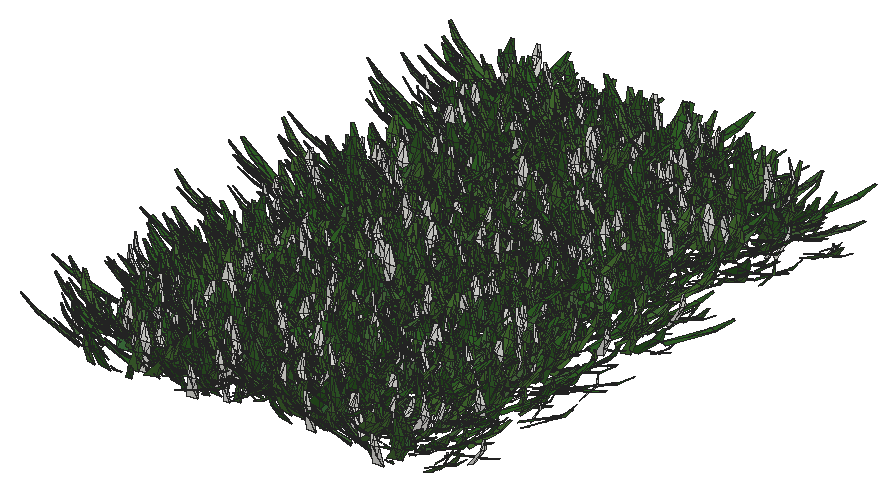
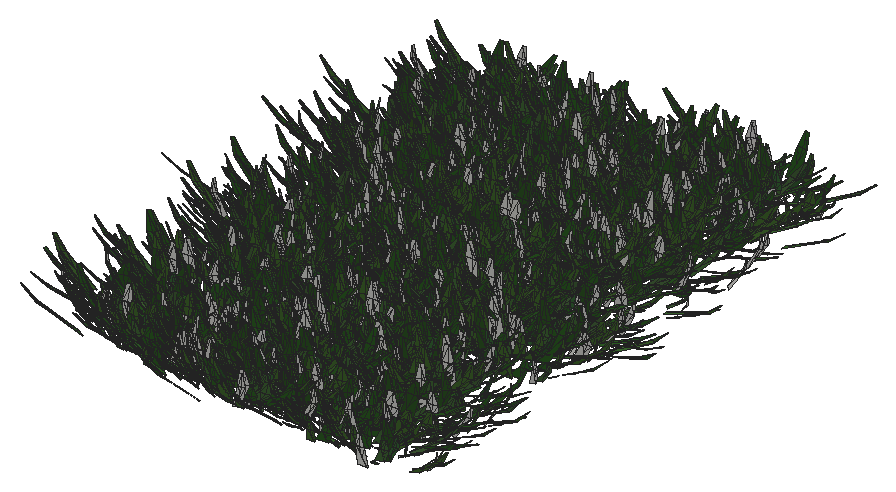
# SketchUp Ruby script. Lengths in inches.
U = 1.inch
M = Sketchup.active_model
def pt(a) = Geom::Point3d.new(a.map { |v| v * U })
def face(e, loops, mat)
  f = e.add_face(loops[0].map { |a| pt(a) })
  loops[1..].each { |l| e.add_face(l.map { |a| pt(a) }).erase! }
  f.material = f.back_material = mat if mat
  f
end
# faces: each face lists its corners as indices into pts; further lists are holes
def faces(e, pts, list, mat = nil) = list.each { |f| face(e, (f[0].is_a?(Array) ? f : [f]).map { |l| l.map { |i| pts[i] } }, mat) }
# xy, xz, yz: faces in a plane at the given z, y or x. An outline is a flat list of corners, or four numbers for a rectangle; further outlines are holes
def ring(l) = l.size == 4 ? [[l[0], l[1]], [l[2], l[1]], [l[2], l[3]], [l[0], l[3]]] : l.each_slice(2).to_a
def flat(e, list, mat, &to3) = list.each { |f| face(e, (f[0].is_a?(Array) ? f : [f]).map { |l| ring(l).map { |u, v| to3.(u, v) } }, mat) }
def xy(e, z, list, mat = nil) = flat(e, list, mat) { |x, y| [x, y, z] }
def xz(e, y, list, mat = nil) = flat(e, list, mat) { |x, z| [x, y, z] }
def yz(e, x, list, mat = nil) = flat(e, list, mat) { |y, z| [x, y, z] }
def lines(e, pts, list) = list.each { |a, b| e.add_line(pt(pts[a]), pt(pts[b])) }
# prism: a flat outline (further loops are holes) pulled along v
def prism(e, loops, v, mat = nil)
  f = face(e, loops, mat); d = Geom::Vector3d.new(v.map { |x| x * U })
  f.pushpull(f.normal.samedirection?(d) ? d.length : -d.length)
end
def box(e, o, s, mat = nil) = prism(e, [[o, [o[0] + s[0], o[1], o[2]], [o[0] + s[0], o[1] + s[1], o[2]], [o[0], o[1] + s[1], o[2]]]], [0, 0, s[2]], mat)
def at(x, y, z, deg = 0) = Geom::Transformation.translation(pt([x, y, z])) * Geom::Transformation.rotation(ORIGIN, Z_AXIS, deg.degrees)
def axes(o, x, y, z) = Geom::Transformation.new([*x, 0, *y, 0, *z, 0, *pt(o).to_a, 1])
def part(name) = M.definitions.add(name)
# library, detail: a bought-in or finely detailed component or shape, given as its bounding box
def library(name, o, s) = part(name).tap { |d| box(d.entities, o, s) }
def detail(e, o, s) = box(e.add_group.entities, o, s)
def put(e, d, t, mat = nil) = e.add_instance(d, t).tap { |i| i.material = mat if mat }
def group(e, t, mat = nil) = e.add_group.tap { |g| g.transformation = t; g.material = mat if mat }.entities
root = M.entities
M.materials.add("Material82").color = [68, 110, 58]
M.materials.add("Material83").color = [48, 90, 38]
M.materials.add("Material84").color = [68, 110, 48]
M.materials.add("Material85").color = [48, 90, 48]
M.materials.add("Material86").color = [58, 110, 58]
M.materials.add("Material87").color = [58, 90, 38]
M.materials.add("Material88").color = [68, 100, 58]
M.materials.add("Material89").color = [48, 100, 38]
c1 = part("grass00")
p = [[-0.6875,0.15,0],[-0.56,0.08,5.52],[-0.04,0.03,2.76],[0.48,-0.02,0],[0.35,-0.02,5.52],[-0.1,-0.14,5.52],
  [-0.12,0.65,8.37],[-0.42,0.65,8.37]]
faces(c1.entities,p,[[0,1,2,3],[3,2,4],[1,5,2],[5,4,2],[1,6,5],[4,5,6],[7,6,1]])
c2 = part("Group16\#1")
put(c2.entities,c1,axes([1.44,-0.61,-0.01],[0.05352,0.12609,0],[-0.10704,0.04543,0.07239],[0.06664,-0.02828,0.11628]),"Material85")
put(c2.entities,c1,axes([0.76,-0.15,-0.01],[0.04676,0.24062,0],[-0.23162,0.04501,0.06642],[0.0652,-0.01267,0.23595]),"Material82")
put(c2.entities,c1,axes([0.79,0.01,-0.01],[-0.00606,0.34651,0],[-0.34381,-0.00602,0.0432],[0.04319,0.00076,0.34386]))
put(c2.entities,c1,axes([1,0.23,-0.01],[-0.07192,0.31144,0],[-0.28722,-0.06632,0.1236],[0.12043,0.02781,0.29478]),"Material84")
put(c2.entities,c1,axes([1.66,0.77,-0.01],[-0.13828,0.29651,0],[-0.21551,-0.1005,0.22471],[0.20365,0.09498,0.23779]),"Material89")
put(c2.entities,c1,axes([0.6875,0.52,-0.01],[-0.18126,0.24051,0],[-0.22746,-0.17142,0.09788],[0.07817,0.05891,0.28481]),"Material84")
put(c2.entities,c1,axes([0.68,0.78,-0.01],[-0.215,0.18688,0],[-0.12385,-0.14248,0.21334],[0.13995,0.16101,0.18878]),"Material82")
put(c2.entities,c1,axes([0.56,1,-0.01],[-0.13756,0.07624,0],[-0.06159,-0.11112,0.0927],[0.04494,0.08108,0.12705]),"Material84")
put(c2.entities,c1,axes([0.2,0.64,-0.01],[-0.23729,0.07254,0],[-0.05711,-0.18681,0.153],[0.04473,0.14632,0.19535]),"Material89")
put(c2.entities,c1,axes([0.0625,0.72,-0.01],[-0.28874,0.02525,0],[-0.02179,-0.24916,0.14647],[0.01276,0.14591,0.25012]),"Material82")
put(c2.entities,c1,axes([-0.08,0.62,-0.01],[-0.34089,-0.04187,0],[0.03255,-0.26504,0.216],[-0.02633,0.21439,0.26703]),"Material89")
put(c2.entities,c1,axes([-0.34,0.98,-0.01],[-0.14314,-0.0493,0],[0.04397,-0.12769,0.06843],[-0.02228,0.0647,0.13505]),"Material89")
put(c2.entities,c1,axes([-0.87,1.45,-0.01],[-0.23488,-0.14114,0],[0.13761,-0.22901,0.06087],[-0.03135,0.05217,0.26717]))
put(c2.entities,c1,axes([-0.72,0.77,-0.01],[-0.14208,-0.13251,0],[0.07209,-0.0773,0.16301],[-0.11118,0.11922,0.1057]),"Material89")
put(c2.entities,c1,axes([-0.62,0.43,-0.01],[-0.14845,-0.21203,0],[0.18654,-0.13061,0.12304],[-0.10079,0.07057,0.22772]),"Material82")
put(c2.entities,c1,axes([-0.68,0.29,-0.01],[-0.13639,-0.32136,0],[0.31723,-0.13464,0.05579],[-0.05136,0.0218,0.34462]),"Material83")
put(c2.entities,c1,axes([-0.64,0.125,-0.01],[-0.0458,-0.23569,0],[0.22124,-0.043,0.08276],[-0.08124,0.01579,0.22538]),"Material86")
put(c2.entities,c1,axes([-1.6,-0.03,-0.01],[0.00576,-0.32897,0],[0.27526,0.00482,0.18018],[-0.18015,-0.00315,0.2753]),"Material84")
put(c2.entities,c1,axes([-1.36,-0.31,-0.01],[0.05718,-0.24765,0],[0.18172,0.04196,0.17267],[-0.16825,-0.03885,0.1865]),"Material89")
put(c2.entities,c1,axes([-1.54,-0.72,-0.01],[0.06537,-0.14017,0],[0.13555,0.06321,0.03939],[-0.0357,-0.01665,0.14956]))
put(c2.entities,c1,axes([-1.19,-0.9,-0.01],[0.09597,-0.12735,0],[0.11214,0.08451,0.07557],[-0.06035,-0.04548,0.14042]),"Material88")
put(c2.entities,c1,axes([-0.47,-0.54,-0.01],[0.11588,-0.10072,0],[0.0618,0.0711,0.12124],[-0.07953,-0.0915,0.0942]))
put(c2.entities,c1,axes([-0.47,-0.84,-0.01],[0.11927,-0.0661,0],[0.06603,0.11913,0.00646],[-0.00313,-0.00565,0.13621]),"Material84")
put(c2.entities,c1,axes([-0.38,-1.24,-0.01],[0.28037,-0.08571,0],[0.0618,0.20215,0.20315],[-0.05939,-0.19428,0.21139]),"Material88")
put(c2.entities,c1,axes([-0.06,-0.66,-0.01],[0.22719,-0.01987,0],[0.01247,0.14255,0.17758],[-0.01547,-0.17691,0.1431]),"Material87")
put(c2.entities,c1,axes([0.11,-0.89,-0.01],[0.14882,0.01828,0],[-0.01058,0.08611,0.12229],[0.01491,-0.12138,0.08676]),"Material85")
put(c2.entities,c1,axes([0.25,-0.72,-0.01],[0.20481,0.07053,0],[-0.06206,0.18022,0.10291],[0.03351,-0.0973,0.1906]),"Material85")
put(c2.entities,c1,axes([0.85,-1.42,-0.01],[0.16481,0.09904,0],[-0.09472,0.15762,0.05616],[0.02893,-0.04814,0.18389]),"Material84")
put(c2.entities,c1,axes([1.01,-1.09,-0.01],[0.21858,0.20385,0],[-0.17495,0.1876,0.15339],[0.10462,-0.11218,0.25652]),"Material89")
put(c2.entities,c1,axes([1.01,-0.71,-0.01],[0.08733,0.12473,0],[-0.06445,0.04512,0.13037],[0.1068,-0.07477,0.07867]),"Material85")
c3 = part("Group15\#1")
put(c3.entities,c2,at(0,0,0))
c4 = part("3darcstudiotree_grass00\#1")
put(c4.entities,c3,at(0,0,0))
put(root,c4,axes([1826.34,333.52,-34.17],[0.25601,-1.60576,0],[3.7655,0.09337,-0.00515],[0.03185,0.00079,1.75106]))
put(root,c4,axes([1825.33,340.01,-34.17],[3.21046,-0.42194,0],[1.31397,1.55496,-0.01535],[0.02427,0.02872,1.5577]))
put(root,c4,axes([1825.35,312.04,-34.17],[-1.88352,1.24088,0],[-3.53635,-0.83485,-0.03562],[-0.13641,-0.0322,1.37892]))
put(root,c4,axes([1826.07,283.93,-34.17],[0.35251,-1.39793,0],[3.51175,0.13773,-0.03727],[0.24286,0.00952,1.73202]))
put(root,c4,axes([1826.34,289.67,-34.17],[-3.43821,0.20499,0],[-0.69374,-1.80975,-0.03474],[-0.02131,-0.0556,1.42794]))
put(root,c4,axes([1825.4,298.68,-34.17],[-0.07716,1.61232,0],[-4.08051,-0.03037,-0.05443],[-0.27918,-0.00208,1.56933]))
put(root,c4,axes([1826.95,320.22,-34.17],[1.28288,-1.22527,0],[4.05082,0.65965,-0.04448],[0.2416,0.03934,1.93016]))
put(root,c4,axes([1827.22,328.61,-34.17],[-0.2981,-1.54731,0],[4.18924,-0.12553,-0.05563],[0.33136,-0.00993,1.88098]))
put(root,c4,axes([1827.06,317.46,-34.17],[-0.54088,1.62044,0],[-3.31155,-0.17191,-0.03263],[-0.19335,-0.01004,1.49628]))
put(root,c4,axes([1827.25,315.92,-34.17],[3.70566,-0.42814,0],[1.15173,1.5504,-0.01036],[0.01836,0.02471,1.93559]))
put(root,c4,axes([1827.75,281.24,-34.17],[2.92691,-1.3802,0],[3.11862,1.02859,-0.02296],[0.10607,0.03499,1.8355]))
put(root,c4,axes([1828.3125,338.09,-34.17],[-3.14741,0.41412,0],[-1.12782,-1.33315,-0.01591],[-0.02767,-0.03271,1.46774]))
put(root,c4,axes([1827.55,335.22,-34.17],[-0.97344,1.33602,0],[-4.5066,-0.51069,-0.06106],[-0.24596,-0.02787,1.47293]))
put(root,c4,axes([1827.37,304.44,-34.17],[4.64499,-0.27977,0],[0.53132,1.372,-0.02943],[0.02555,0.06597,1.51666]))
put(root,c4,axes([1828.82,302.05,-34.17],[-0.18207,-1.50592,0],[4.09357,-0.07698,-0.05646],[0.28834,-0.00542,1.57058]))
put(root,c4,axes([1827.49,291.67,-34.17],[2.47814,1.17598,0],[-3.14029,1.02922,-0.05468],[-0.21842,0.07159,1.58958]))
put(root,c4,axes([1827.46,313.96,-34.17],[4.42055,0.62646,0],[-1.4719,1.61538,-0.03831],[-0.06085,0.06679,1.53223]))
put(root,c4,axes([1827.99,330.81,-34.17],[4.51641,-0.1704,0],[0.33815,1.39393,-0.00501],[0.00291,0.012,1.62495]))
put(root,c4,axes([1827.6875,293.85,-34.17],[2.33395,1.59128,0],[-3.69314,0.84246,-0.02506],[-0.12399,0.02828,1.82822]))
put(root,c4,axes([1828.27,285.62,-34.17],[3.72841,-0.11021,0],[0.34874,1.83494,-0.00347],[0.00143,0.00753,1.92949]))
put(root,c4,axes([1829.27,326.92,-34.17],[-2.15234,1.14546,0],[-3.3995,-0.99347,-0.05517],[-0.2418,-0.07066,1.72999]))
put(root,c4,axes([1828.57,300.64,-34.17],[2.3917,1.38211,0],[-2.775,0.74686,-0.01403],[-0.09111,0.02452,1.97952]))
put(root,c4,axes([1828.67,309.31,-34.17],[3.05644,0.96272,0],[-2.54771,1.25799,-0.04015],[-0.1144,0.05649,1.39698]))
put(root,c4,axes([1829.22,296.33,-34.17],[0.44258,1.4547,0],[-3.4051,0.16112,-0.01784],[-0.12417,0.00588,1.80168]))
put(root,c4,axes([1830.86,323.88,-34.17],[-1.45799,-1.43911,0],[3.11235,-0.49041,-0.01431],[0.09188,-0.01448,1.73701]))
put(root,c4,axes([1831.01,283.47,-34.17],[-2.77273,1.25915,0],[-2.61353,-0.89509,-0.01448],[-0.05898,-0.0202,1.39954]))
put(root,c4,axes([1831.98,285,-34.17],[-3.67224,-0.62774,0],[1.3268,-1.20717,-0.04544],[0.10775,-0.09803,1.4908]))
put(root,c4,axes([1832.23,317.6,-34.17],[-4.47177,0.4092,0],[-0.80597,-1.36984,-0.03599],[-0.04373,-0.07433,1.43677]))
put(root,c4,axes([1831.62,295.9,-34.17],[-3.07968,1.30519,0],[-3.32937,-1.22181,-0.01383],[-0.04412,-0.01619,1.48532]))
put(root,c4,axes([1832.39,339.19,-34.17],[-3.54635,0.32604,0],[-1.06041,-1.79388,-0.06463],[-0.05576,-0.09432,1.33032]))
put(root,c4,axes([1831.16,307.32,-34.17],[3.91717,0.58785,0],[-1.40512,1.45623,-0.01203],[-0.02325,0.0241,1.60927]))
put(root,c4,axes([1833.02,302.46,-34.17],[-1.04981,-1.26066,0],[3.51989,-0.45588,-0.02104],[0.10484,-0.01358,1.45661]))
put(root,c4,axes([1832.29,299.02,-34.17],[3.15172,-0.92963,0],[2.70365,1.42561,-0.02614],[0.06865,0.0362,1.48366]))
put(root,c4,axes([1833.06,305.26,-34.17],[-4.56421,0.17831,0],[-0.33265,-1.32435,-0.0174],[-0.0117,-0.04658,1.72585]))
put(root,c4,axes([1833.55,330.95,-34.17],[-3.08784,-0.53374,0],[1.78756,-1.6084,-0.00176],[0.00414,-0.00372,1.95594]))
put(root,c4,axes([1832.6,291.37,-34.17],[-2.14552,1.35971,0],[-3.80804,-0.93454,-0.04897],[-0.2422,-0.05944,1.9584]))
put(root,c4,axes([1832.0625,288.08,-34.17],[3.03533,0.518,0],[-1.31858,1.2017,-0.02703],[-0.08286,0.07551,1.9211]))
put(root,c4,axes([1833.9,313.28,-34.17],[-2.79081,-0.68685,0],[2.20267,-1.39196,-0.00523],[0.01654,-0.01045,1.86317]))
put(root,c4,axes([1834.04,316.69,-34.17],[-3.42781,-0.73376,0],[1.91044,-1.38806,-0.04387],[0.11882,-0.08633,1.70431]))
put(root,c4,axes([1833.34,289.42,-34.17],[-3.41152,0.77464,0],[-2.34689,-1.60751,-0.0199],[-0.0471,-0.03226,1.67187]))
put(root,c4,axes([1832.35,312.07,-34.17],[1.53269,1.16919,0],[-3.90157,0.79546,-0.03477],[-0.15934,0.03249,1.69826]))
put(root,c4,axes([1833.64,300.03,-34.17],[-2.82754,1.11661,0],[-2.90837,-1.14544,-0.05526],[-0.21558,-0.0849,1.69871]))
put(root,c4,axes([1833.65,293.44,-34.17],[2.39859,-1.38317,0],[2.89597,0.78107,-0.02882],[0.1286,0.03468,1.42183]))
put(root,c4,axes([1834.08,337.85,-34.17],[0.37671,-1.60669,0],[3.58296,0.13066,-0.04487],[0.23434,0.00855,1.41449]))
put(root,c4,axes([1834.48,336.35,-34.17],[-4.41181,-0.09171,0],[0.23476,-1.75641,-0.0488],[0.01273,-0.09527,1.65721]))
put(root,c4,axes([1834.35,281.67,-34.17],[-3.47293,0.19496,0],[-0.50842,-1.40863,-0.03826],[-0.03299,-0.09141,1.65468]))
put(root,c4,axes([1834.91,332.71,-34.17],[-4.2727,-0.29638,0],[0.78575,-1.76178,-0.04722],[0.03378,-0.07573,1.40384]))
put(root,c4,axes([1833.5625,328.23,-34.17],[-0.9668,1.66725,0],[-3.92404,-0.3539,-0.0233],[-0.11915,-0.01075,1.58282]))
put(root,c4,axes([1833.61,309.55,-34.17],[3.78841,0.96012,0],[-2.55963,1.5708,-0.03131],[-0.07104,0.04359,1.48921]))
put(root,c4,axes([1833.86,322.55,-34.17],[2.7139,1.45109,0],[-3.63417,1.0571,-0.05484],[-0.17137,0.04985,1.31443]))
put(root,c4,axes([1834.42,320.54,-34.17],[3.41186,0.04199,0],[-0.11049,1.39641,-0.01718],[-0.0038,0.04797,1.88076]))
put(root,c4,axes([1836.49,299.01,-34.17],[-3.09292,-0.92086,0],[2.57207,-1.3436,-0.01411],[0.04505,-0.02353,1.69584]))
put(root,c4,axes([1834.64,326.3125,-34.17],[0.1551,1.54916,0],[-4.73746,0.07377,-0.04149],[-0.18002,0.0028,1.54325]))
put(root,c4,axes([1836.67,317.79,-34.17],[0.67498,-1.80639,0],[4.18251,0.24307,-0.00777],[0.03281,0.00191,1.3523]))
put(root,c4,axes([1836.83,313.77,-34.17],[-0.75947,-1.30953,0],[4.19896,-0.37875,-0.04627],[0.26037,-0.02349,1.86363]))
put(root,c4,axes([1836.875,300.08,-34.17],[-4.1346,0.13575,0],[-0.2838,-1.34436,-0.02559],[-0.01617,-0.0766,1.95328]))
put(root,c4,axes([1837.65,311.39,-34.17],[1.00092,-1.32759,0],[4.42574,0.51896,-0.06029],[0.29852,0.035,1.78762]))
put(root,c4,axes([1837.35,332.57,-34.17],[2.10537,-1.23806,0],[3.71835,0.98344,-0.05795],[0.27877,0.07373,1.94389]))
put(root,c4,axes([1836.7,287.45,-34.17],[3.79547,0.16316,0],[-0.37027,1.33962,-0.03498],[-0.02197,0.07948,1.48455]))
put(root,c4,axes([1837.54,306.96,-34.17],[-3.00276,0.99555,0],[-2.11915,-0.9941,-0.00081],[-0.00373,-0.00175,1.76997]))
put(root,c4,axes([1838.66,325.16,-34.17],[-0.04764,-1.42757,0],[4.50476,-0.02338,-0.00745],[0.04284,-0.00022,1.94284]))
put(root,c4,axes([1837.36,283.19,-34.17],[0.27257,1.5962,0],[-3.57048,0.09483,-0.04154],[-0.28788,0.00765,1.86323]))
put(root,c4,axes([1838.8,320.39,-34.17],[-4.51182,-0.35471,0],[0.87439,-1.72977,-0.01918],[0.02129,-0.04212,1.90358]))
put(root,c4,axes([1837.57,327.35,-34.17],[2.9902,-0.77103,0],[1.83544,1.10708,-0.045],[0.13449,0.08112,1.37282]))
put(root,c4,axes([1838.85,305.3,-34.17],[0.52861,-1.48035,0],[4.44113,0.24665,-0.00524],[0.03043,0.00169,1.97007]))
put(root,c4,axes([1837.15,294.74,-34.17],[1.62026,1.14881,0],[-2.90984,0.63829,-0.00131],[-0.00892,0.00196,1.9458]))
put(root,c4,axes([1838.17,285.1875,-34.17],[-3.07094,0.93295,0],[-2.23562,-1.14452,-0.00087],[-0.00325,-0.00166,1.68429]))
put(root,c4,axes([1839.21,291.54,-34.17],[-1.32818,-1.26932,0],[4.11875,-0.67029,-0.01762],[0.07227,-0.01176,1.48208]))
put(root,c4,axes([1837.31,289.16,-34.17],[3.48613,0.95688,0],[-2.23612,1.26704,-0.01513],[-0.04219,0.02391,1.43215]))
put(root,c4,axes([1838.39,322.25,-34.17],[3.73229,-0.67208,0],[1.78653,1.54305,-0.05401],[0.10032,0.08665,1.44188]))
put(root,c4,axes([1840.04,335.35,-34.17],[-3.64932,-0.7532,0],[1.94147,-1.463,-0.05348],[0.14522,-0.10943,1.83786]))
put(root,c4,axes([1838.74,309.52,-34.17],[4.39358,-0.14103,0],[0.35283,1.70956,-0.02372],[0.00876,0.04243,1.48337]))
put(root,c4,axes([1840.23,336.93,-34.17],[-4.22243,0.41861,0],[-0.86072,-1.35028,-0.03206],[-0.04838,-0.0759,1.63785]))
put(root,c4,axes([1839.25,328.72,-34.17],[2.4549,0.99675,0],[-3.14112,1.20322,-0.03466],[-0.14383,0.05509,1.89896]))
put(root,c4,axes([1839.29,315.6,-34.17],[3.48474,0.89145,0],[-2.45497,1.49256,-0.05832],[-0.13986,0.08503,1.48992]))
put(root,c4,axes([1839.83,331.39,-34.17],[-0.03901,1.43427,0],[-3.74587,-0.01585,-0.03184],[-0.19446,-0.00082,1.71482]))
put(root,c4,axes([1840.21,303.07,-34.17],[-1.95042,1.47202,0],[-4.16072,-0.85742,-0.06253],[-0.2988,-0.06158,1.89715]))
put(root,c4,axes([1840.11,296.46,-34.17],[3.54296,-0.10072,0],[0.24357,1.33252,-0.00836],[0.00467,0.02557,1.97523]))
put(root,c4,axes([1842.31,313.82,-34.17],[-3.58618,-0.76762,0],[2.12856,-1.54662,-0.04044],[0.10752,-0.07813,1.86421]))
put(root,c4,axes([1840.33,339.32,-34.17],[3.38325,1.26435,0],[-2.73925,1.14001,-0.00751],[-0.0314,0.01307,1.8142]))
put(root,c4,axes([1842.58,309.27,-34.17],[-3.71376,-0.4791,0],[1.06109,-1.27925,-0.035],[0.07367,-0.08882,1.73222]))
put(root,c4,axes([1843.13,329.42,-34.17],[-3.76687,-0.82913,0],[2.27178,-1.60524,-0.0179],[0.04066,-0.02873,1.62858]))
put(root,c4,axes([1842.3,291.75,-34.17],[-3.28554,0.84585,0],[-2.43757,-1.4726,-0.04574],[-0.1384,-0.08361,1.85022]))
put(root,c4,axes([1843.04,290.41,-34.17],[0.43132,-1.66774,0],[3.95027,0.1589,-0.00761],[0.04938,0.00199,1.94156]))
put(root,c4,axes([1843.3,317.49,-34.17],[-3.03865,-1.23581,0],[2.76731,-1.05827,-0.04714],[0.18592,-0.0711,1.58733]))
put(root,c4,axes([1841.89,286.78,-34.17],[4.71636,-0.1967,0],[0.48906,1.82382,-0.02611],[0.01545,0.05763,1.96192]))
put(root,c4,axes([1842.98,320.03,-34.17],[-3.07129,1.23004,0],[-2.90171,-1.12685,-0.02428],[-0.07533,-0.02925,1.32917]))
put(root,c4,axes([1843.89,294.77,-34.17],[-3.14124,-0.52931,0],[1.80451,-1.66556,-0.04539],[0.09971,-0.09203,1.92461]))
put(root,c4,axes([1842.61,338.31,-34.17],[4.37264,-0.16186,0],[0.38997,1.63854,-0.03728],[0.02119,0.08905,1.90298]))
put(root,c4,axes([1842.96,332.74,-34.17],[4.22982,-0.69798,0],[1.45654,1.37281,-0.04818],[0.09708,0.0915,1.47658]))
put(root,c4,axes([1843.22,331.78,-34.17],[3.5272,-0.10967,0],[0.36977,1.84972,-0.03935],[0.01267,0.0634,1.44542]))
put(root,c4,axes([1843.95,324.05,-34.17],[2.22522,-0.98382,0],[3.26699,1.14926,-0.04874],[0.15967,0.05617,1.44038]))
put(root,c4,axes([1843.16,298.49,-34.17],[4.40761,-0.00182,0],[0.00468,1.76466,-0.04894],[0.00022,0.08123,1.41164]))
put(root,c4,axes([1843.33,339.18,-34.17],[3.37216,0.16863,0],[-0.47809,1.48691,-0.01144],[-0.0086,0.02673,1.7012]))
put(root,c4,axes([1845.05,316.68,-34.17],[-3.1255,-0.93872,0],[2.35839,-1.22127,-0.01582],[0.04515,-0.02338,1.37394]))
put(root,c4,axes([1844.01,312.24,-34.17],[-2.15998,1.50569,0],[-3.5128,-0.78375,-0.02589],[-0.10439,-0.02329,1.40149]))
put(root,c4,axes([1844.49,335.6,-34.17],[2.50422,-1.12718,0],[2.64209,0.91293,-0.00209],[0.0092,0.00318,1.54397]))
put(root,c4,axes([1844.64,327.24,-34.17],[-3.79899,1.04858,0],[-2.13311,-1.20197,-0.01309],[-0.05055,-0.02848,1.87779]))
put(root,c4,axes([1845.3125,297.02,-34.17],[-0.77442,-1.59147,0],[3.42237,-0.25901,-0.00431],[0.02185,-0.00165,1.34772]))
put(root,c4,axes([1845.59,283.77,-34.17],[-1.56215,-1.16443,0],[3.47638,-0.72535,-0.0302],[0.1517,-0.03165,1.67548]))
put(root,c4,axes([1845.68,302.51,-34.17],[0.16922,-1.40325,0],[3.56749,0.06691,-0.0123],[0.08099,0.00152,1.7643]))
put(root,c4,axes([1844.5,306.82,-34.17],[3.21803,0.34517,0],[-1.06694,1.54707,-0.02379],[-0.03071,0.04453,1.49895]))
put(root,c4,axes([1844.26,300.53,-34.17],[1.18275,1.22871,0],[-4.35683,0.65227,-0.02635],[-0.11985,0.01794,1.69955]))
put(root,c4,axes([1845.93,322.41,-34.17],[-4.55654,0.30056,0],[-0.72952,-1.72007,-0.00717],[-0.00538,-0.01268,1.50735]))
put(root,c4,axes([1845.42,305.49,-34.17],[2.66801,-0.76193,0],[2.24823,1.2244,-0.04376],[0.15596,0.08494,1.7457]))
put(root,c4,axes([1847.51,313.06,-34.17],[-2.4386,-1.43306,0],[3.07254,-0.81318,-0.00883],[0.05033,-0.01332,1.90461]))
put(root,c4,axes([1847.88,331.49,-34.17],[-2.69612,-1.17454,0],[3.29179,-1.17522,-0.01753],[0.05781,-0.02064,1.48083]))
put(root,c4,axes([1845.84,285.37,-34.17],[-0.169,1.77802,0],[-4.32571,-0.06395,-0.00219],[-0.00941,-0.00014,1.39308]))
put(root,c4,axes([1848.08,289.02,-34.17],[-3.83813,-1.06248,0],[2.06139,-1.15817,-0.02484],[0.08815,-0.04953,1.66133]))
put(root,c4,axes([1847.77,325.34,-34.17],[-4.08007,0.11151,0],[-0.22831,-1.29918,-0.01842],[-0.00694,-0.03947,1.34789]))
put(root,c4,axes([1848.25,283.58,-34.17],[-3.13096,0.65051,0],[-1.62991,-1.22011,-0.01732],[-0.0588,-0.04402,1.90951]))
put(root,c4,axes([1849.46,335.92,-34.17],[-1.34356,-1.54381,0],[4.22745,-0.57221,-0.00214],[0.01038,-0.00141,1.72072]))
put(root,c4,axes([1847.52,291.125,-34.17],[3.83567,0.80348,0],[-1.71741,1.27513,-0.04207],[-0.13622,0.10114,1.89419]))
put(root,c4,axes([1847.94,307.22,-34.17],[2.14752,1.24419,0],[-2.84206,0.76295,-0.02533],[-0.12904,0.03464,1.58831]))
put(root,c4,axes([1848.55,329.55,-34.17],[4.00755,-0.76372,0],[1.77132,1.44561,-0.00312],[0.00773,0.00631,1.73901]))
put(root,c4,axes([1848.25,300.73,-34.17],[0.92286,1.78615,0],[-4.03148,0.32396,-0.0503],[-0.25163,0.02022,1.57458]))
put(root,c4,axes([1848.58,315.79,-34.17],[-1.5079,1.48015,0],[-3.78766,-0.60014,-0.02547],[-0.10708,-0.01697,1.38631]))
put(root,c4,axes([1849.63,297.77,-34.17],[0.88426,-1.72062,0],[4.38154,0.35021,-0.041],[0.21175,0.01693,1.76588]))
put(root,c4,axes([1848.45,293.66,-34.17],[4.1439,0.48612,0],[-1.21296,1.60815,-0.03162],[-0.038,0.05038,1.3441]))
put(root,c4,axes([1848.31,308.79,-34.17],[2.12924,1.06786,0],[-3.55371,1.10206,-0.01217],[-0.05143,0.01595,1.82194]))
put(root,c4,axes([1849.88,284.69,-34.17],[1.5808,-1.43275,0],[3.65536,0.62726,-0.04597],[0.19603,0.03364,1.38947]))
put(root,c4,axes([1850.77,288,-34.17],[-4.27451,-0.64112,0],[1.27307,-1.32012,-0.04106],[0.09351,-0.09696,1.71966]))
put(root,c4,axes([1850.69,332.92,-34.17],[-3.75297,0.08152,0],[-0.23562,-1.68719,-0.02509],[-0.00578,-0.04142,1.34616]))
put(root,c4,axes([1850.6875,338.3,-34.17],[-3.08585,0.75112,0],[-1.75968,-1.12437,-0.03387],[-0.09597,-0.06132,1.3548]))
put(root,c4,axes([1851.34,323.26,-34.17],[-0.74737,-1.75822,0],[4.00395,-0.2647,-0.02808],[0.1526,-0.01009,1.67665]))
put(root,c4,axes([1850.58,304.49,-34.17],[2.37533,-1.57622,0],[3.03149,0.71052,-0.0411],[0.20378,0.04776,1.52451]))
put(root,c4,axes([1849.78,317.97,-34.17],[3.22242,0.46316,0],[-1.61234,1.7447,-0.03532],[-0.06153,0.06658,1.79519]))
put(root,c4,axes([1850.27,312.34,-34.17],[0.53134,1.4221,0],[-3.42638,0.19911,-0.04131],[-0.21204,0.01232,1.34689]))
put(root,c4,axes([1850.76,303.55,-34.17],[3.9417,-1.03975,0],[1.84996,1.09076,-0.03191],[0.12762,0.07525,1.79443]))
put(root,c4,axes([1851.14,296.27,-34.17],[3.56947,-0.45549,0],[1.31887,1.60745,-0.01717],[0.02449,0.02985,1.48777]))
put(root,c4,axes([1851.22,319.66,-34.17],[0.55525,1.71346,0],[-3.482,0.17549,-0.04145],[-0.30813,0.01553,1.97198]))
put(root,c4,axes([1850.97,326.65,-34.17],[3.66484,0.89609,0],[-2.00603,1.27601,-0.03504],[-0.12347,0.07854,1.90819]))
put(root,c4,axes([1853.1875,289.59,-34.17],[-1.10349,-1.4395,0],[4.41957,-0.52692,-0.03772],[0.14279,-0.01702,1.36861]))
put(root,c4,axes([1852.98,319.5,-34.17],[-2.20687,1.14075,0],[-3.09016,-0.92978,-0.05103],[-0.23957,-0.07208,1.72023]))
put(root,c4,axes([1853.45,331.53,-34.17],[-3.32366,1.12138,0],[-2.70082,-1.24501,-0.05065],[-0.15287,-0.07047,1.44592]))
put(root,c4,axes([1854.53,316.28,-34.17],[-2.7638,-1.30283,0],[3.13183,-1.03331,-0.01878],[0.07913,-0.02611,1.68146]))
put(root,c4,axes([1854.76,309,-34.17],[-3.16827,-0.67396,0],[1.62868,-1.19079,-0.04409],[0.1208,-0.08832,1.48398]))
put(root,c4,axes([1854.51,317.34,-34.17],[-4.1698,0.79339,0],[-1.666,-1.36181,-0.02532],[-0.06287,-0.05139,1.64221]))
put(root,c4,axes([1853.48,337.66,-34.17],[3.81533,0.48086,0],[-1.13696,1.40304,-0.03842],[-0.0798,0.09848,1.90991]))
put(root,c4,axes([1854.09,302.06,-34.17],[3.77642,-0.7823,0],[1.66108,1.24712,-0.02304],[0.07142,0.05362,1.78453]))
put(root,c4,axes([1855.62,329.27,-34.17],[0.63263,-1.77026,0],[4.09912,0.22783,-0.02402],[0.14113,0.00784,1.84088]))
put(root,c4,axes([1855.76,293.54,-34.17],[-4.44839,0.03138,0],[-0.07411,-1.6342,-0.01042],[-0.00109,-0.02408,1.82123]))
put(root,c4,axes([1855.74,282.67,-34.17],[-3.4085,0.44598,0],[-1.18576,-1.40948,-0.04681],[-0.08042,-0.0956,1.53984]))
put(root,c4,axes([1854.5,292.31,-34.17],[3.54482,0.3991,0],[-1.20365,1.66273,-0.00872],[-0.01104,0.01525,1.51538]))
put(root,c4,axes([1855.125,322.3,-34.17],[-0.28998,1.73456,0],[-3.34694,-0.08702,-0.03816],[-0.29536,-0.00768,1.95014]))
put(root,c4,axes([1854.35,287.11,-34.17],[3.41397,1.21641,0],[-2.3032,1.00536,-0.00582],[-0.0237,0.01035,1.56404]))
put(root,c4,axes([1854.47,298.54,-34.17],[2.93721,1.2592,0],[-3.10849,1.12772,-0.033],[-0.144,0.05224,1.87715]))
put(root,c4,axes([1856.63,300.11,-34.17],[-1.1478,-1.40641,0],[4.093,-0.51953,-0.0477],[0.19511,-0.02477,1.385]))
put(root,c4,axes([1857.02,285.97,-34.17],[-2.49924,-1.08664,0],[2.82442,-1.01033,-0.0539],[0.19999,-0.07154,1.43163]))
put(root,c4,axes([1855.41,305.5,-34.17],[2.93445,0.88211,0],[-2.13254,1.10335,-0.01463],[-0.05848,0.03025,1.73802]))
put(root,c4,axes([1855.53,297,-34.17],[3.48566,0.55514,0],[-1.55719,1.52067,-0.03343],[-0.07577,0.07399,1.88641]))
put(root,c4,axes([1855.99,335.54,-34.17],[-0.15322,1.4871,0],[-3.57108,-0.05722,-0.03031],[-0.19833,-0.00318,1.75443]))
put(root,c4,axes([1855.69,314.39,-34.17],[3.31433,0.47754,0],[-1.51472,1.63504,-0.04863],[-0.07862,0.08486,1.5585]))
put(root,c4,axes([1856.92,334.13,-34.17],[-3.94658,0.83198,0],[-2.08533,-1.53849,-0.02635],[-0.05206,-0.03841,1.3895]))
put(root,c4,axes([1855.54,326.65,-34.17],[2.20824,1.44568,0],[-4.06639,0.96604,-0.01693],[-0.06521,0.01549,1.59984]))
put(root,c4,axes([1856.27,310.95,-34.17],[4.53975,0.53985,0],[-1.08694,1.4216,-0.04516],[-0.08333,0.10898,1.80387]))
